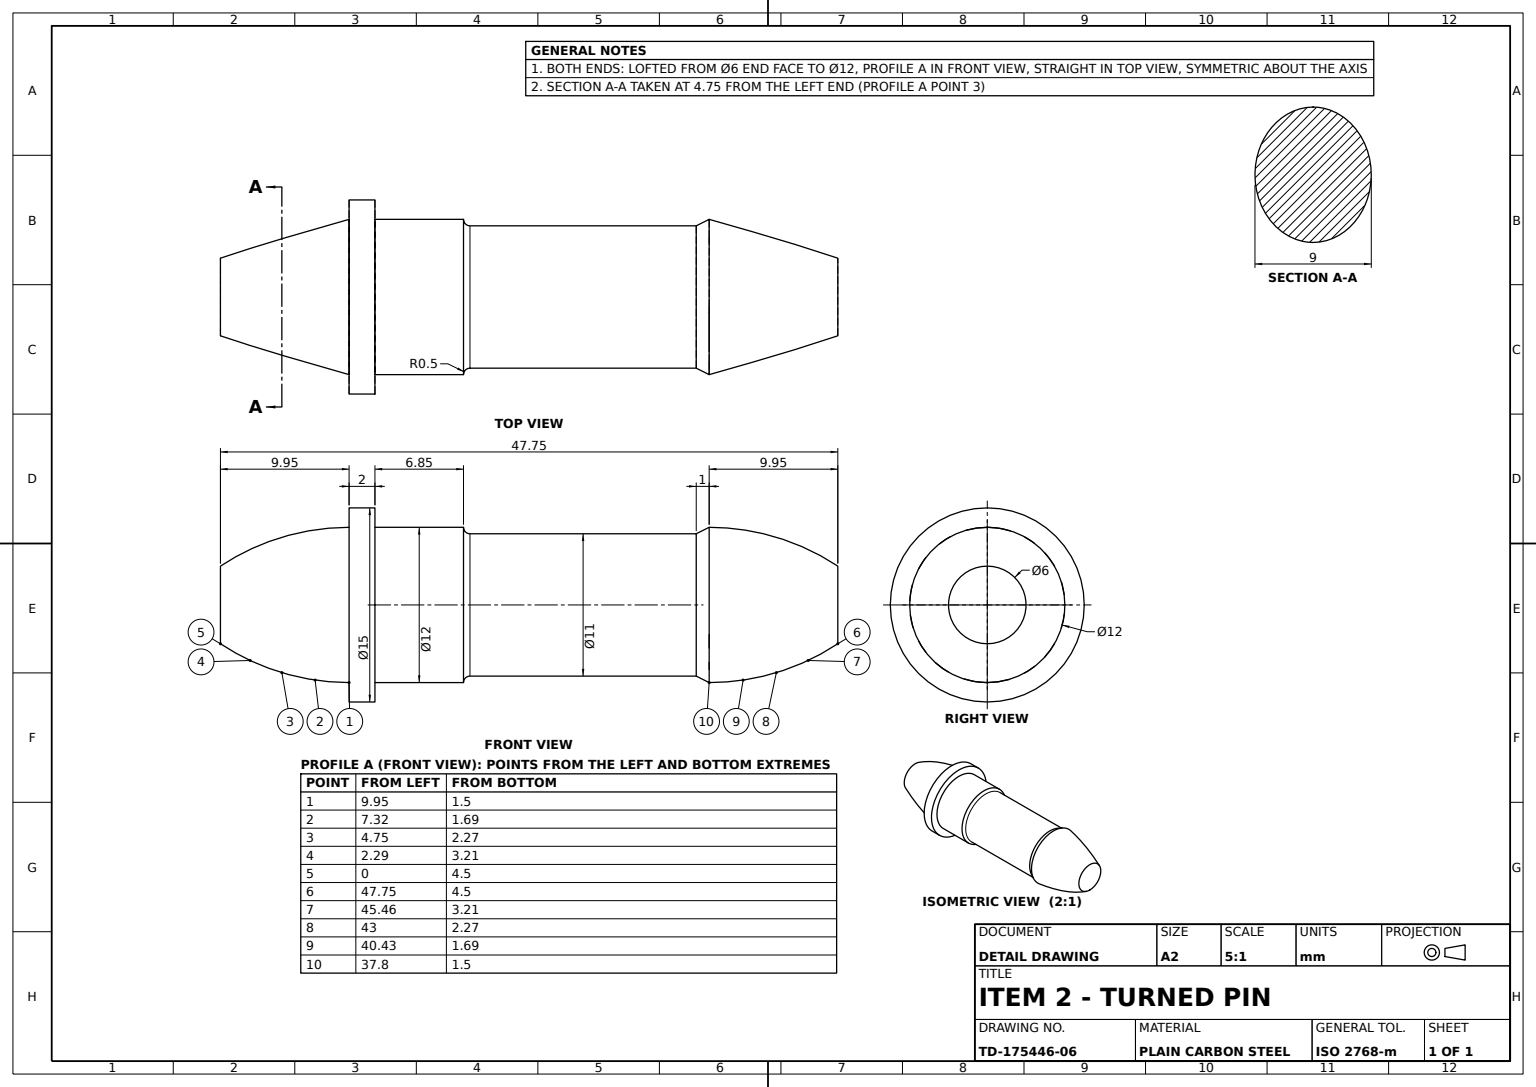
ISO-10303-21;
HEADER;
FILE_DESCRIPTION((''),'2;1');
FILE_NAME('','',(''),(''),'','','');
FILE_SCHEMA(('AUTOMOTIVE_DESIGN'));
ENDSEC;
DATA;
#1=APPLICATION_CONTEXT('');
#2=PRODUCT_CONTEXT('',#1,'mechanical');
#3=PRODUCT('','','',(#2));
#4=PRODUCT_DEFINITION_FORMATION('','',#3);
#5=PRODUCT_DEFINITION_CONTEXT('',#1,'design');
#6=PRODUCT_DEFINITION('','',#4,#5);
#7=PRODUCT_DEFINITION_SHAPE('','',#6);
#8=(LENGTH_UNIT()NAMED_UNIT(*)SI_UNIT(.MILLI.,.METRE.));
#9=(NAMED_UNIT(*)PLANE_ANGLE_UNIT()SI_UNIT($,.RADIAN.));
#10=(NAMED_UNIT(*)SI_UNIT($,.STERADIAN.)SOLID_ANGLE_UNIT());
#11=UNCERTAINTY_MEASURE_WITH_UNIT(LENGTH_MEASURE(1.E-05),#8,'distance_accuracy_value','');
#12=(GEOMETRIC_REPRESENTATION_CONTEXT(3)GLOBAL_UNCERTAINTY_ASSIGNED_CONTEXT((#11))GLOBAL_UNIT_ASSIGNED_CONTEXT((#8,#9,#10))REPRESENTATION_CONTEXT('',''));
#13=CARTESIAN_POINT('',(0.,11.95,7.5));
#14=VERTEX_POINT('',#13);
#15=CARTESIAN_POINT('',(0.,11.95,-7.5));
#16=VERTEX_POINT('',#15);
#17=CARTESIAN_POINT('',(0.,11.95,0.));
#18=DIRECTION('',(0.,1.,0.));
#19=DIRECTION('',(0.,0.,1.));
#20=AXIS2_PLACEMENT_3D('',#17,#18,#19);
#21=CIRCLE('',#20,7.5);
#22=EDGE_CURVE('',#14,#16,#21,.T.);
#23=ORIENTED_EDGE('',*,*,#22,.F.);
#24=CARTESIAN_POINT('',(0.,9.95,7.5));
#25=VERTEX_POINT('',#24);
#26=DIRECTION('',(0.,-1.,0.));
#27=VECTOR('',#26,1000.);
#28=LINE('',#13,#27);
#29=EDGE_CURVE('',#14,#25,#28,.T.);
#30=ORIENTED_EDGE('',*,*,#29,.T.);
#31=CARTESIAN_POINT('',(0.,9.95,-7.5));
#32=VERTEX_POINT('',#31);
#33=CARTESIAN_POINT('',(0.,9.95,0.));
#34=AXIS2_PLACEMENT_3D('',#33,#18,#19);
#35=CIRCLE('',#34,7.5);
#36=EDGE_CURVE('',#25,#32,#35,.T.);
#37=ORIENTED_EDGE('',*,*,#36,.T.);
#38=LINE('',#15,#27);
#39=EDGE_CURVE('',#16,#32,#38,.T.);
#40=ORIENTED_EDGE('',*,*,#39,.F.);
#41=EDGE_LOOP('',(#23,#30,#37,#40));
#42=FACE_OUTER_BOUND('',#41,.T.);
#43=DIRECTION('',(0.,0.,-1.));
#44=AXIS2_PLACEMENT_3D('',#17,#26,#43);
#45=CYLINDRICAL_SURFACE('',#44,7.5);
#46=ADVANCED_FACE('',(#42),#45,.T.);
#47=CARTESIAN_POINT('',(0.,11.95,6.));
#48=VERTEX_POINT('',#47);
#49=CARTESIAN_POINT('',(0.,11.95,-6.));
#50=VERTEX_POINT('',#49);
#51=CIRCLE('',#20,6.);
#52=EDGE_CURVE('',#48,#50,#51,.T.);
#53=ORIENTED_EDGE('',*,*,#52,.F.);
#54=EDGE_CURVE('',#50,#48,#51,.T.);
#55=ORIENTED_EDGE('',*,*,#54,.F.);
#56=EDGE_LOOP('',(#53,#55));
#57=FACE_BOUND('',#56,.T.);
#58=ORIENTED_EDGE('',*,*,#22,.T.);
#59=EDGE_CURVE('',#16,#14,#21,.T.);
#60=ORIENTED_EDGE('',*,*,#59,.T.);
#61=EDGE_LOOP('',(#58,#60));
#62=FACE_OUTER_BOUND('',#61,.T.);
#63=PLANE('',#20);
#64=ADVANCED_FACE('',(#57,#62),#63,.T.);
#65=CARTESIAN_POINT('',(0.,36.8,5.5));
#66=VERTEX_POINT('',#65);
#67=CARTESIAN_POINT('',(0.,19.3,5.5));
#68=VERTEX_POINT('',#67);
#69=LINE('',#65,#27);
#70=EDGE_CURVE('',#66,#68,#69,.T.);
#71=ORIENTED_EDGE('',*,*,#70,.T.);
#72=CARTESIAN_POINT('',(0.,19.3,-5.5));
#73=VERTEX_POINT('',#72);
#74=CARTESIAN_POINT('',(0.,19.3,0.));
#75=AXIS2_PLACEMENT_3D('',#74,#18,#19);
#76=CIRCLE('',#75,5.5);
#77=EDGE_CURVE('',#68,#73,#76,.T.);
#78=ORIENTED_EDGE('',*,*,#77,.T.);
#79=CARTESIAN_POINT('',(0.,36.8,-5.5));
#80=VERTEX_POINT('',#79);
#81=LINE('',#79,#27);
#82=EDGE_CURVE('',#80,#73,#81,.T.);
#83=ORIENTED_EDGE('',*,*,#82,.F.);
#84=CARTESIAN_POINT('',(0.,36.8,0.));
#85=AXIS2_PLACEMENT_3D('',#84,#18,#19);
#86=CIRCLE('',#85,5.5);
#87=EDGE_CURVE('',#66,#80,#86,.T.);
#88=ORIENTED_EDGE('',*,*,#87,.F.);
#89=EDGE_LOOP('',(#71,#78,#83,#88));
#90=FACE_OUTER_BOUND('',#89,.T.);
#91=AXIS2_PLACEMENT_3D('',#84,#26,#43);
#92=CYLINDRICAL_SURFACE('',#91,5.5);
#93=ADVANCED_FACE('',(#90),#92,.T.);
#94=ORIENTED_EDGE('',*,*,#82,.T.);
#95=EDGE_CURVE('',#73,#68,#76,.T.);
#96=ORIENTED_EDGE('',*,*,#95,.T.);
#97=ORIENTED_EDGE('',*,*,#70,.F.);
#98=EDGE_CURVE('',#80,#66,#86,.T.);
#99=ORIENTED_EDGE('',*,*,#98,.F.);
#100=EDGE_LOOP('',(#94,#96,#97,#99));
#101=FACE_OUTER_BOUND('',#100,.T.);
#102=ADVANCED_FACE('',(#101),#92,.T.);
#103=CARTESIAN_POINT('',(0.,18.8,6.));
#104=VERTEX_POINT('',#103);
#105=CARTESIAN_POINT('',(0.,19.3,6.));
#106=DIRECTION('',(-1.,0.,0.));
#107=AXIS2_PLACEMENT_3D('',#105,#106,#19);
#108=CIRCLE('',#107,0.5);
#109=EDGE_CURVE('',#68,#104,#108,.T.);
#110=ORIENTED_EDGE('',*,*,#109,.F.);
#111=ORIENTED_EDGE('',*,*,#95,.F.);
#112=CARTESIAN_POINT('',(0.,18.8,-6.));
#113=VERTEX_POINT('',#112);
#114=CARTESIAN_POINT('',(0.,19.3,-6.));
#115=DIRECTION('',(1.,0.,0.));
#116=AXIS2_PLACEMENT_3D('',#114,#115,#43);
#117=CIRCLE('',#116,0.5);
#118=EDGE_CURVE('',#73,#113,#117,.T.);
#119=ORIENTED_EDGE('',*,*,#118,.T.);
#120=CARTESIAN_POINT('',(0.,18.8,0.));
#121=AXIS2_PLACEMENT_3D('',#120,#18,#19);
#122=CIRCLE('',#121,6.);
#123=EDGE_CURVE('',#113,#104,#122,.T.);
#124=ORIENTED_EDGE('',*,*,#123,.T.);
#125=EDGE_LOOP('',(#110,#111,#119,#124));
#126=FACE_OUTER_BOUND('',#125,.T.);
#127=TOROIDAL_SURFACE('',#75,6.,0.5);
#128=ADVANCED_FACE('',(#126),#127,.F.);
#129=CARTESIAN_POINT('',(-3.,0.,0.));
#130=VERTEX_POINT('',#129);
#131=CARTESIAN_POINT('',(3.,0.,0.));
#132=VERTEX_POINT('',#131);
#133=CARTESIAN_POINT('',(0.,0.,0.));
#134=AXIS2_PLACEMENT_3D('',#133,#18,#19);
#135=CIRCLE('',#134,3.);
#136=EDGE_CURVE('',#130,#132,#135,.T.);
#137=ORIENTED_EDGE('',*,*,#136,.T.);
#138=CARTESIAN_POINT('',(6.,9.95,0.));
#139=VERTEX_POINT('',#138);
#140=CARTESIAN_POINT('',(6.000025,6.410631,0.));
#141=CARTESIAN_POINT('',(4.95646,2.949474,0.));
#142=B_SPLINE_CURVE_WITH_KNOTS('',3,(#138,#140,#141,#131),.UNSPECIFIED.,.F.,.F.,(4,4),(0.,1.),.UNSPECIFIED.);
#143=EDGE_CURVE('',#139,#132,#142,.T.);
#144=ORIENTED_EDGE('',*,*,#143,.F.);
#145=CARTESIAN_POINT('',(-6.,9.95,0.));
#146=VERTEX_POINT('',#145);
#147=CIRCLE('',#34,6.);
#148=EDGE_CURVE('',#146,#139,#147,.T.);
#149=ORIENTED_EDGE('',*,*,#148,.F.);
#150=CARTESIAN_POINT('',(-6.000025,6.410631,0.));
#151=CARTESIAN_POINT('',(-4.95646,2.949474,0.));
#152=B_SPLINE_CURVE_WITH_KNOTS('',3,(#145,#150,#151,#129),.UNSPECIFIED.,.F.,.F.,(4,4),(0.,1.),.UNSPECIFIED.);
#153=EDGE_CURVE('',#146,#130,#152,.T.);
#154=ORIENTED_EDGE('',*,*,#153,.T.);
#155=EDGE_LOOP('',(#137,#144,#149,#154));
#156=FACE_OUTER_BOUND('',#155,.T.);
#157=CARTESIAN_POINT('',(-6.,9.95,-0.785398));
#158=CARTESIAN_POINT('',(-6.000025,6.410631,-0.654498));
#159=CARTESIAN_POINT('',(-4.95646,2.949474,-0.523599));
#160=CARTESIAN_POINT('',(-3.,0.,-0.392699));
#161=CARTESIAN_POINT('',(-5.687979,9.95,-2.355842));
#162=CARTESIAN_POINT('',(-5.677499,6.410631,-1.963227));
#163=CARTESIAN_POINT('',(-4.688654,2.949474,-1.570612));
#164=CARTESIAN_POINT('',(-2.84397,0.,-1.177998));
#165=CARTESIAN_POINT('',(-4.353184,9.95,-4.353257));
#166=CARTESIAN_POINT('',(-4.33079,6.410631,-3.627716));
#167=CARTESIAN_POINT('',(-3.574621,2.949474,-2.902175));
#168=CARTESIAN_POINT('',(-2.176574,0.,-2.176634));
#169=CARTESIAN_POINT('',(-2.356027,9.95,-5.687748));
#170=CARTESIAN_POINT('',(-2.338359,6.410631,-4.739794));
#171=CARTESIAN_POINT('',(-1.929344,2.949474,-3.791841));
#172=CARTESIAN_POINT('',(-1.177994,0.,-2.843888));
#173=CARTESIAN_POINT('',(0.,9.95,-6.156445));
#174=CARTESIAN_POINT('',(0.,6.410631,-5.130367));
#175=CARTESIAN_POINT('',(0.,2.949474,-4.10429));
#176=CARTESIAN_POINT('',(0.,0.,-3.078212));
#177=CARTESIAN_POINT('',(2.356027,9.95,-5.687748));
#178=CARTESIAN_POINT('',(2.338359,6.410631,-4.739794));
#179=CARTESIAN_POINT('',(1.929344,2.949474,-3.791841));
#180=CARTESIAN_POINT('',(1.177994,0.,-2.843888));
#181=CARTESIAN_POINT('',(4.353184,9.95,-4.353257));
#182=CARTESIAN_POINT('',(4.33079,6.410631,-3.627716));
#183=CARTESIAN_POINT('',(3.574621,2.949474,-2.902175));
#184=CARTESIAN_POINT('',(2.176574,0.,-2.176634));
#185=CARTESIAN_POINT('',(5.687979,9.95,-2.355842));
#186=CARTESIAN_POINT('',(5.677499,6.410631,-1.963227));
#187=CARTESIAN_POINT('',(4.688654,2.949474,-1.570612));
#188=CARTESIAN_POINT('',(2.84397,0.,-1.177998));
#189=CARTESIAN_POINT('',(6.,9.95,-0.785398));
#190=CARTESIAN_POINT('',(6.000025,6.410631,-0.654498));
#191=CARTESIAN_POINT('',(4.95646,2.949474,-0.523599));
#192=CARTESIAN_POINT('',(3.,0.,-0.392699));
#193=CARTESIAN_POINT('',(6.,9.95,0.785398));
#194=CARTESIAN_POINT('',(6.000025,6.410631,0.654498));
#195=CARTESIAN_POINT('',(4.95646,2.949474,0.523599));
#196=CARTESIAN_POINT('',(3.,0.,0.392699));
#197=CARTESIAN_POINT('',(5.687979,9.95,2.355842));
#198=CARTESIAN_POINT('',(5.677499,6.410631,1.963227));
#199=CARTESIAN_POINT('',(4.688654,2.949474,1.570612));
#200=CARTESIAN_POINT('',(2.84397,0.,1.177998));
#201=CARTESIAN_POINT('',(4.353184,9.95,4.353257));
#202=CARTESIAN_POINT('',(4.33079,6.410631,3.627716));
#203=CARTESIAN_POINT('',(3.574621,2.949474,2.902175));
#204=CARTESIAN_POINT('',(2.176574,0.,2.176634));
#205=CARTESIAN_POINT('',(2.356027,9.95,5.687748));
#206=CARTESIAN_POINT('',(2.338359,6.410631,4.739794));
#207=CARTESIAN_POINT('',(1.929344,2.949474,3.791841));
#208=CARTESIAN_POINT('',(1.177994,0.,2.843888));
#209=CARTESIAN_POINT('',(0.,9.95,6.156445));
#210=CARTESIAN_POINT('',(0.,6.410631,5.130367));
#211=CARTESIAN_POINT('',(0.,2.949474,4.10429));
#212=CARTESIAN_POINT('',(0.,0.,3.078212));
#213=CARTESIAN_POINT('',(-2.356027,9.95,5.687748));
#214=CARTESIAN_POINT('',(-2.338359,6.410631,4.739794));
#215=CARTESIAN_POINT('',(-1.929344,2.949474,3.791841));
#216=CARTESIAN_POINT('',(-1.177994,0.,2.843888));
#217=CARTESIAN_POINT('',(-4.353184,9.95,4.353257));
#218=CARTESIAN_POINT('',(-4.33079,6.410631,3.627716));
#219=CARTESIAN_POINT('',(-3.574621,2.949474,2.902175));
#220=CARTESIAN_POINT('',(-2.176574,0.,2.176634));
#221=CARTESIAN_POINT('',(-5.687979,9.95,2.355842));
#222=CARTESIAN_POINT('',(-5.677499,6.410631,1.963227));
#223=CARTESIAN_POINT('',(-4.688654,2.949474,1.570612));
#224=CARTESIAN_POINT('',(-2.84397,0.,1.177998));
#225=CARTESIAN_POINT('',(-6.,9.95,0.785398));
#226=CARTESIAN_POINT('',(-6.000025,6.410631,0.654498));
#227=CARTESIAN_POINT('',(-4.95646,2.949474,0.523599));
#228=CARTESIAN_POINT('',(-3.,0.,0.392699));
#229=B_SPLINE_SURFACE_WITH_KNOTS('',3,3,((#145,#150,#151,#129),(#157,#158,#159,#160),(#161,#162,#163,#164),(#165,#166,#167,#168),(#169,#170,#171,#172),(#173,#174,#175,#176),(#177,#178,#179,#180),(#181,#182,#183,#184),(#185,#186,#187,#188),(#189,#190,#191,#192),(#193,#194,#195,#196),(#197,#198,#199,#200),(#201,#202,#203,#204),(#205,#206,#207,#208),(#209,#210,#211,#212),(#213,#214,#215,#216),(#217,#218,#219,#220),(#221,#222,#223,#224),(#225,#226,#227,#228),(#145,#150,#151,#129)),.UNSPECIFIED.,.T.,.F.,.F.,(4,1,1,1,1,1,1,1,2,1,1,1,1,1,1,1,4),(4,4),(0.,0.0625,0.125,0.1875,0.25,0.3125,0.375,0.4375,0.5,0.5625,0.625,0.6875,0.75,0.8125,0.875,0.9375,1.),(0.,1.),.UNSPECIFIED.);
#230=ADVANCED_FACE('',(#156),#229,.T.);
#231=ORIENTED_EDGE('',*,*,#143,.T.);
#232=EDGE_CURVE('',#132,#130,#135,.T.);
#233=ORIENTED_EDGE('',*,*,#232,.T.);
#234=ORIENTED_EDGE('',*,*,#153,.F.);
#235=EDGE_CURVE('',#139,#146,#147,.T.);
#236=ORIENTED_EDGE('',*,*,#235,.F.);
#237=EDGE_LOOP('',(#231,#233,#234,#236));
#238=FACE_OUTER_BOUND('',#237,.T.);
#239=ADVANCED_FACE('',(#238),#229,.T.);
#240=ORIENTED_EDGE('',*,*,#87,.T.);
#241=CARTESIAN_POINT('',(0.,37.800271,-6.000136));
#242=VERTEX_POINT('',#241);
#243=DIRECTION('',(0.,0.894427191,-0.447213595));
#244=VECTOR('',#243,1000.);
#245=LINE('',#79,#244);
#246=EDGE_CURVE('',#80,#242,#245,.T.);
#247=ORIENTED_EDGE('',*,*,#246,.T.);
#248=CARTESIAN_POINT('',(6.,37.8,0.));
#249=VERTEX_POINT('',#248);
#250=CARTESIAN_POINT('',(6.,37.8,-0.396106));
#251=CARTESIAN_POINT('',(5.96083,37.799345,-0.788083));
#252=CARTESIAN_POINT('',(5.805864,37.799586,-1.563958));
#253=CARTESIAN_POINT('',(5.691379,37.80042,-1.939901));
#254=CARTESIAN_POINT('',(5.466806,37.800439,-2.480886));
#255=CARTESIAN_POINT('',(5.383007,37.800219,-2.657661));
#256=CARTESIAN_POINT('',(5.197439,37.799868,-3.004071));
#257=CARTESIAN_POINT('',(5.09506,37.799736,-3.174509));
#258=CARTESIAN_POINT('',(4.766595,37.799721,-3.66508));
#259=CARTESIAN_POINT('',(4.51867,37.800321,-3.966961));
#260=CARTESIAN_POINT('',(3.96495,37.800289,-4.520413));
#261=CARTESIAN_POINT('',(3.655958,37.79972,-4.773424));
#262=CARTESIAN_POINT('',(3.004636,37.799744,-5.208062));
#263=CARTESIAN_POINT('',(2.660278,37.800276,-5.39254));
#264=CARTESIAN_POINT('',(2.114851,37.800271,-5.618519));
#265=CARTESIAN_POINT('',(1.927546,37.800108,-5.685407));
#266=CARTESIAN_POINT('',(1.551266,37.799856,-5.799254));
#267=CARTESIAN_POINT('',(1.361395,37.799765,-5.846652));
#268=CARTESIAN_POINT('',(0.786699,37.799773,-5.960901));
#269=CARTESIAN_POINT('',(0.395479,37.800271,-6.000136));
#270=B_SPLINE_CURVE_WITH_KNOTS('',3,(#248,#250,#251,#252,#253,#254,#255,#256,#257,#258,#259,#260,#261,#262,#263,#264,#265,#266,#267,#268,#269,#241),.UNSPECIFIED.,.F.,.F.,(4,2,2,2,2,2,2,2,2,2,4),(0.,0.001181769,0.002363539,0.002954424,0.003545308,0.004727078,0.005908847,0.007090617,0.007681501,0.008272386,0.009454155),.UNSPECIFIED.);
#271=EDGE_CURVE('',#249,#242,#270,.T.);
#272=ORIENTED_EDGE('',*,*,#271,.F.);
#273=CARTESIAN_POINT('',(0.,37.800271,6.000136));
#274=VERTEX_POINT('',#273);
#275=CARTESIAN_POINT('',(0.391395,37.800271,6.000136));
#276=CARTESIAN_POINT('',(0.780802,37.799774,5.961961));
#277=CARTESIAN_POINT('',(1.361889,37.799764,5.846609));
#278=CARTESIAN_POINT('',(1.554432,37.799857,5.798398));
#279=CARTESIAN_POINT('',(1.930162,37.80011,5.684511));
#280=CARTESIAN_POINT('',(2.114372,37.80027,5.618651));
#281=CARTESIAN_POINT('',(2.475504,37.800275,5.469161));
#282=CARTESIAN_POINT('',(2.652427,37.800116,5.385529));
#283=CARTESIAN_POINT('',(2.998941,37.799846,5.200386));
#284=CARTESIAN_POINT('',(3.169439,37.799737,5.098235));
#285=CARTESIAN_POINT('',(3.661542,37.799723,4.769396));
#286=CARTESIAN_POINT('',(3.963959,37.800287,4.521289));
#287=CARTESIAN_POINT('',(4.517933,37.800323,3.967811));
#288=CARTESIAN_POINT('',(4.771322,37.799716,3.658773));
#289=CARTESIAN_POINT('',(5.207048,37.799746,3.006486));
#290=CARTESIAN_POINT('',(5.391801,37.800449,2.661952));
#291=CARTESIAN_POINT('',(5.617869,37.800424,2.116788));
#292=CARTESIAN_POINT('',(5.684858,37.800172,1.92931));
#293=CARTESIAN_POINT('',(5.798959,37.799718,1.552159));
#294=CARTESIAN_POINT('',(5.846407,37.799521,1.361946));
#295=CARTESIAN_POINT('',(5.960742,37.79935,0.786529));
#296=CARTESIAN_POINT('',(6.,37.8,0.396444));
#297=B_SPLINE_CURVE_WITH_KNOTS('',3,(#273,#275,#276,#277,#278,#279,#280,#281,#282,#283,#284,#285,#286,#287,#288,#289,#290,#291,#292,#293,#294,#295,#296,#248),.UNSPECIFIED.,.F.,.F.,(4,2,2,2,2,2,2,2,2,2,2,4),(0.028375947,0.029558724,0.030150113,0.030741502,0.03133289,0.031924279,0.033107057,0.034289834,0.035472612,0.036064,0.036655389,0.037838166),.UNSPECIFIED.);
#298=EDGE_CURVE('',#274,#249,#297,.T.);
#299=ORIENTED_EDGE('',*,*,#298,.F.);
#300=DIRECTION('',(0.,0.894427191,0.447213595));
#301=VECTOR('',#300,1000.);
#302=LINE('',#65,#301);
#303=EDGE_CURVE('',#66,#274,#302,.T.);
#304=ORIENTED_EDGE('',*,*,#303,.F.);
#305=EDGE_LOOP('',(#240,#247,#272,#299,#304));
#306=FACE_OUTER_BOUND('',#305,.T.);
#307=CONICAL_SURFACE('',#85,5.5,0.463647609);
#308=ADVANCED_FACE('',(#306),#307,.T.);
#309=ORIENTED_EDGE('',*,*,#232,.F.);
#310=ORIENTED_EDGE('',*,*,#136,.F.);
#311=EDGE_LOOP('',(#309,#310));
#312=FACE_OUTER_BOUND('',#311,.T.);
#313=PLANE('',#134);
#314=ADVANCED_FACE('',(#312),#313,.F.);
#315=EDGE_CURVE('',#32,#25,#35,.T.);
#316=ORIENTED_EDGE('',*,*,#315,.F.);
#317=ORIENTED_EDGE('',*,*,#36,.F.);
#318=EDGE_LOOP('',(#316,#317));
#319=FACE_OUTER_BOUND('',#318,.T.);
#320=ORIENTED_EDGE('',*,*,#235,.T.);
#321=ORIENTED_EDGE('',*,*,#148,.T.);
#322=EDGE_LOOP('',(#320,#321));
#323=FACE_BOUND('',#322,.T.);
#324=PLANE('',#34);
#325=ADVANCED_FACE('',(#319,#323),#324,.F.);
#326=EDGE_CURVE('',#104,#113,#122,.T.);
#327=ORIENTED_EDGE('',*,*,#326,.T.);
#328=ORIENTED_EDGE('',*,*,#118,.F.);
#329=ORIENTED_EDGE('',*,*,#77,.F.);
#330=ORIENTED_EDGE('',*,*,#109,.T.);
#331=EDGE_LOOP('',(#327,#328,#329,#330));
#332=FACE_OUTER_BOUND('',#331,.T.);
#333=ADVANCED_FACE('',(#332),#127,.F.);
#334=ORIENTED_EDGE('',*,*,#39,.T.);
#335=ORIENTED_EDGE('',*,*,#315,.T.);
#336=ORIENTED_EDGE('',*,*,#29,.F.);
#337=ORIENTED_EDGE('',*,*,#59,.F.);
#338=EDGE_LOOP('',(#334,#335,#336,#337));
#339=FACE_OUTER_BOUND('',#338,.T.);
#340=ADVANCED_FACE('',(#339),#45,.T.);
#341=CARTESIAN_POINT('',(-6.,37.8,0.));
#342=VERTEX_POINT('',#341);
#343=CARTESIAN_POINT('',(-6.,37.8,0.391456));
#344=CARTESIAN_POINT('',(-5.960463,37.799348,0.788981));
#345=CARTESIAN_POINT('',(-5.807334,37.799582,1.557528));
#346=CARTESIAN_POINT('',(-5.694396,37.80041,1.931618));
#347=CARTESIAN_POINT('',(-5.468635,37.800444,2.476975));
#348=CARTESIAN_POINT('',(-5.383433,37.80022,2.65682));
#349=CARTESIAN_POINT('',(-5.197635,37.799868,3.00375));
#350=CARTESIAN_POINT('',(-5.096789,37.799738,3.171649));
#351=CARTESIAN_POINT('',(-4.770991,37.799718,3.659059));
#352=CARTESIAN_POINT('',(-4.522534,37.80032,3.963007));
#353=CARTESIAN_POINT('',(-3.962453,37.80029,4.523));
#354=CARTESIAN_POINT('',(-3.659317,37.799723,4.770807));
#355=CARTESIAN_POINT('',(-3.171758,37.799737,5.096723));
#356=CARTESIAN_POINT('',(-3.003709,37.799843,5.197655));
#357=CARTESIAN_POINT('',(-2.65624,37.800113,5.38367));
#358=CARTESIAN_POINT('',(-2.476492,37.800275,5.468752));
#359=CARTESIAN_POINT('',(-1.931843,37.800267,5.694209));
#360=CARTESIAN_POINT('',(-1.557858,37.799764,5.807368));
#361=CARTESIAN_POINT('',(-0.788514,37.799771,5.960766));
#362=CARTESIAN_POINT('',(-0.391202,37.800271,6.000136));
#363=B_SPLINE_CURVE_WITH_KNOTS('',3,(#341,#343,#344,#345,#346,#347,#348,#349,#350,#351,#352,#353,#354,#355,#356,#357,#358,#359,#360,#361,#362,#273),.UNSPECIFIED.,.F.,.F.,(4,2,2,2,2,2,2,2,2,2,4),(0.01891838,0.020100576,0.021282772,0.02187387,0.022464967,0.023647163,0.024829359,0.025420457,0.026011555,0.027193751,0.028375947),.UNSPECIFIED.);
#364=EDGE_CURVE('',#342,#274,#363,.T.);
#365=ORIENTED_EDGE('',*,*,#364,.F.);
#366=CARTESIAN_POINT('',(-0.3959,37.800271,-6.000136));
#367=CARTESIAN_POINT('',(-0.785591,37.799774,-5.961089));
#368=CARTESIAN_POINT('',(-1.361251,37.799765,-5.846696));
#369=CARTESIAN_POINT('',(-1.551646,37.799856,-5.799178));
#370=CARTESIAN_POINT('',(-1.929362,37.800109,-5.684818));
#371=CARTESIAN_POINT('',(-2.116584,37.800272,-5.617856));
#372=CARTESIAN_POINT('',(-2.66111,37.800274,-5.392084));
#373=CARTESIAN_POINT('',(-3.005742,37.799743,-5.20751));
#374=CARTESIAN_POINT('',(-3.658823,37.799722,-4.771325));
#375=CARTESIAN_POINT('',(-3.967566,37.800293,-4.51811));
#376=CARTESIAN_POINT('',(-4.520806,37.800317,-3.964512));
#377=CARTESIAN_POINT('',(-4.769144,37.799717,-3.661947));
#378=CARTESIAN_POINT('',(-5.208416,37.799746,-3.004524));
#379=CARTESIAN_POINT('',(-5.394292,37.800455,-2.656526));
#380=CARTESIAN_POINT('',(-5.618576,37.800421,-2.114788));
#381=CARTESIAN_POINT('',(-5.68446,37.800173,-1.930438));
#382=CARTESIAN_POINT('',(-5.798408,37.79972,-1.554165));
#383=CARTESIAN_POINT('',(-5.846642,37.79952,-1.361163));
#384=CARTESIAN_POINT('',(-5.961681,37.79935,-0.78099));
#385=CARTESIAN_POINT('',(-6.,37.8,-0.391731));
#386=B_SPLINE_CURVE_WITH_KNOTS('',3,(#241,#366,#367,#368,#369,#370,#371,#372,#373,#374,#375,#376,#377,#378,#379,#380,#381,#382,#383,#384,#385,#341),.UNSPECIFIED.,.F.,.F.,(4,2,2,2,2,2,2,2,2,2,4),(0.009454155,0.010637183,0.011228698,0.011820212,0.01300324,0.014186268,0.015369296,0.016552324,0.017143838,0.017735352,0.01891838),.UNSPECIFIED.);
#387=EDGE_CURVE('',#242,#342,#386,.T.);
#388=ORIENTED_EDGE('',*,*,#387,.F.);
#389=ORIENTED_EDGE('',*,*,#246,.F.);
#390=ORIENTED_EDGE('',*,*,#98,.T.);
#391=ORIENTED_EDGE('',*,*,#303,.T.);
#392=EDGE_LOOP('',(#365,#388,#389,#390,#391));
#393=FACE_OUTER_BOUND('',#392,.T.);
#394=ADVANCED_FACE('',(#393),#307,.T.);
#395=CARTESIAN_POINT('',(3.,47.75,0.));
#396=VERTEX_POINT('',#395);
#397=CARTESIAN_POINT('',(-3.,47.75,0.));
#398=VERTEX_POINT('',#397);
#399=CARTESIAN_POINT('',(0.,47.75,0.));
#400=AXIS2_PLACEMENT_3D('',#399,#18,#19);
#401=CIRCLE('',#400,3.);
#402=EDGE_CURVE('',#396,#398,#401,.T.);
#403=ORIENTED_EDGE('',*,*,#402,.T.);
#404=EDGE_CURVE('',#398,#396,#401,.T.);
#405=ORIENTED_EDGE('',*,*,#404,.T.);
#406=EDGE_LOOP('',(#403,#405));
#407=FACE_OUTER_BOUND('',#406,.T.);
#408=PLANE('',#400);
#409=ADVANCED_FACE('',(#407),#408,.T.);
#410=ORIENTED_EDGE('',*,*,#402,.F.);
#411=CARTESIAN_POINT('',(4.95646,44.800526,0.));
#412=CARTESIAN_POINT('',(6.000025,41.339369,0.));
#413=B_SPLINE_CURVE_WITH_KNOTS('',3,(#395,#411,#412,#248),.UNSPECIFIED.,.F.,.F.,(4,4),(0.,1.),.UNSPECIFIED.);
#414=EDGE_CURVE('',#396,#249,#413,.T.);
#415=ORIENTED_EDGE('',*,*,#414,.T.);
#416=ORIENTED_EDGE('',*,*,#271,.T.);
#417=ORIENTED_EDGE('',*,*,#387,.T.);
#418=CARTESIAN_POINT('',(-4.95646,44.800526,0.));
#419=CARTESIAN_POINT('',(-6.000025,41.339369,0.));
#420=B_SPLINE_CURVE_WITH_KNOTS('',3,(#397,#418,#419,#341),.UNSPECIFIED.,.F.,.F.,(4,4),(0.,1.),.UNSPECIFIED.);
#421=EDGE_CURVE('',#398,#342,#420,.T.);
#422=ORIENTED_EDGE('',*,*,#421,.F.);
#423=EDGE_LOOP('',(#410,#415,#416,#417,#422));
#424=FACE_OUTER_BOUND('',#423,.T.);
#425=CARTESIAN_POINT('',(-6.,37.764606,0.));
#426=CARTESIAN_POINT('',(-6.,37.729213,0.));
#427=CARTESIAN_POINT('',(-5.999999,37.693819,0.));
#428=CARTESIAN_POINT('',(-3.,47.75,-0.392699));
#429=CARTESIAN_POINT('',(-4.95646,44.800526,-0.523599));
#430=CARTESIAN_POINT('',(-6.000025,41.339369,-0.654498));
#431=CARTESIAN_POINT('',(-6.,37.8,-0.785398));
#432=CARTESIAN_POINT('',(-6.,37.764606,-0.786707));
#433=CARTESIAN_POINT('',(-6.,37.729213,-0.788016));
#434=CARTESIAN_POINT('',(-5.999999,37.693819,-0.789325));
#435=CARTESIAN_POINT('',(-2.84397,47.75,-1.177998));
#436=CARTESIAN_POINT('',(-4.688654,44.800526,-1.570612));
#437=CARTESIAN_POINT('',(-5.677499,41.339369,-1.963227));
#438=CARTESIAN_POINT('',(-5.687979,37.8,-2.355842));
#439=CARTESIAN_POINT('',(-5.688083,37.764606,-2.359768));
#440=CARTESIAN_POINT('',(-5.688188,37.729213,-2.363694));
#441=CARTESIAN_POINT('',(-5.688293,37.693819,-2.36762));
#442=CARTESIAN_POINT('',(-2.176574,47.75,-2.176634));
#443=CARTESIAN_POINT('',(-3.574621,44.800526,-2.902175));
#444=CARTESIAN_POINT('',(-4.33079,41.339369,-3.627716));
#445=CARTESIAN_POINT('',(-4.353184,37.8,-4.353257));
#446=CARTESIAN_POINT('',(-4.353408,37.764606,-4.360512));
#447=CARTESIAN_POINT('',(-4.353632,37.729213,-4.367767));
#448=CARTESIAN_POINT('',(-4.353856,37.693819,-4.375023));
#449=CARTESIAN_POINT('',(-1.177994,47.75,-2.843888));
#450=CARTESIAN_POINT('',(-1.929344,44.800526,-3.791841));
#451=CARTESIAN_POINT('',(-2.338359,41.339369,-4.739794));
#452=CARTESIAN_POINT('',(-2.356027,37.8,-5.687748));
#453=CARTESIAN_POINT('',(-2.356204,37.764606,-5.697227));
#454=CARTESIAN_POINT('',(-2.35638,37.729213,-5.706707));
#455=CARTESIAN_POINT('',(-2.356557,37.693819,-5.716186));
#456=CARTESIAN_POINT('',(0.,47.75,-3.078212));
#457=CARTESIAN_POINT('',(0.,44.800526,-4.10429));
#458=CARTESIAN_POINT('',(0.,41.339369,-5.130367));
#459=CARTESIAN_POINT('',(0.,37.8,-6.156445));
#460=CARTESIAN_POINT('',(0.,37.764606,-6.166705));
#461=CARTESIAN_POINT('',(0.,37.729213,-6.176966));
#462=CARTESIAN_POINT('',(0.,37.693819,-6.187227));
#463=CARTESIAN_POINT('',(1.177994,47.75,-2.843888));
#464=CARTESIAN_POINT('',(1.929344,44.800526,-3.791841));
#465=CARTESIAN_POINT('',(2.338359,41.339369,-4.739794));
#466=CARTESIAN_POINT('',(2.356027,37.8,-5.687748));
#467=CARTESIAN_POINT('',(2.356204,37.764606,-5.697227));
#468=CARTESIAN_POINT('',(2.35638,37.729213,-5.706707));
#469=CARTESIAN_POINT('',(2.356557,37.693819,-5.716186));
#470=CARTESIAN_POINT('',(2.176574,47.75,-2.176634));
#471=CARTESIAN_POINT('',(3.574621,44.800526,-2.902175));
#472=CARTESIAN_POINT('',(4.33079,41.339369,-3.627716));
#473=CARTESIAN_POINT('',(4.353184,37.8,-4.353257));
#474=CARTESIAN_POINT('',(4.353408,37.764606,-4.360512));
#475=CARTESIAN_POINT('',(4.353632,37.729213,-4.367767));
#476=CARTESIAN_POINT('',(4.353856,37.693819,-4.375023));
#477=CARTESIAN_POINT('',(2.84397,47.75,-1.177998));
#478=CARTESIAN_POINT('',(4.688654,44.800526,-1.570612));
#479=CARTESIAN_POINT('',(5.677499,41.339369,-1.963227));
#480=CARTESIAN_POINT('',(5.687979,37.8,-2.355842));
#481=CARTESIAN_POINT('',(5.688083,37.764606,-2.359768));
#482=CARTESIAN_POINT('',(5.688188,37.729213,-2.363694));
#483=CARTESIAN_POINT('',(5.688293,37.693819,-2.36762));
#484=CARTESIAN_POINT('',(3.,47.75,-0.392699));
#485=CARTESIAN_POINT('',(4.95646,44.800526,-0.523599));
#486=CARTESIAN_POINT('',(6.000025,41.339369,-0.654498));
#487=CARTESIAN_POINT('',(6.,37.8,-0.785398));
#488=CARTESIAN_POINT('',(6.,37.764606,-0.786707));
#489=CARTESIAN_POINT('',(6.,37.729213,-0.788016));
#490=CARTESIAN_POINT('',(5.999999,37.693819,-0.789325));
#491=CARTESIAN_POINT('',(3.,47.75,0.392699));
#492=CARTESIAN_POINT('',(4.95646,44.800526,0.523599));
#493=CARTESIAN_POINT('',(6.000025,41.339369,0.654498));
#494=CARTESIAN_POINT('',(6.,37.8,0.785398));
#495=CARTESIAN_POINT('',(6.,37.764606,0.786707));
#496=CARTESIAN_POINT('',(6.,37.729213,0.788016));
#497=CARTESIAN_POINT('',(5.999999,37.693819,0.789325));
#498=CARTESIAN_POINT('',(2.84397,47.75,1.177998));
#499=CARTESIAN_POINT('',(4.688654,44.800526,1.570612));
#500=CARTESIAN_POINT('',(5.677499,41.339369,1.963227));
#501=CARTESIAN_POINT('',(5.687979,37.8,2.355842));
#502=CARTESIAN_POINT('',(5.688083,37.764606,2.359768));
#503=CARTESIAN_POINT('',(5.688188,37.729213,2.363694));
#504=CARTESIAN_POINT('',(5.688293,37.693819,2.36762));
#505=CARTESIAN_POINT('',(2.176574,47.75,2.176634));
#506=CARTESIAN_POINT('',(3.574621,44.800526,2.902175));
#507=CARTESIAN_POINT('',(4.33079,41.339369,3.627716));
#508=CARTESIAN_POINT('',(4.353184,37.8,4.353257));
#509=CARTESIAN_POINT('',(4.353408,37.764606,4.360512));
#510=CARTESIAN_POINT('',(4.353632,37.729213,4.367767));
#511=CARTESIAN_POINT('',(4.353856,37.693819,4.375023));
#512=CARTESIAN_POINT('',(1.177994,47.75,2.843888));
#513=CARTESIAN_POINT('',(1.929344,44.800526,3.791841));
#514=CARTESIAN_POINT('',(2.338359,41.339369,4.739794));
#515=CARTESIAN_POINT('',(2.356027,37.8,5.687748));
#516=CARTESIAN_POINT('',(2.356204,37.764606,5.697227));
#517=CARTESIAN_POINT('',(2.35638,37.729213,5.706707));
#518=CARTESIAN_POINT('',(2.356557,37.693819,5.716186));
#519=CARTESIAN_POINT('',(0.,47.75,3.078212));
#520=CARTESIAN_POINT('',(0.,44.800526,4.10429));
#521=CARTESIAN_POINT('',(0.,41.339369,5.130367));
#522=CARTESIAN_POINT('',(0.,37.8,6.156445));
#523=CARTESIAN_POINT('',(0.,37.764606,6.166705));
#524=CARTESIAN_POINT('',(0.,37.729213,6.176966));
#525=CARTESIAN_POINT('',(0.,37.693819,6.187227));
#526=CARTESIAN_POINT('',(-1.177994,47.75,2.843888));
#527=CARTESIAN_POINT('',(-1.929344,44.800526,3.791841));
#528=CARTESIAN_POINT('',(-2.338359,41.339369,4.739794));
#529=CARTESIAN_POINT('',(-2.356027,37.8,5.687748));
#530=CARTESIAN_POINT('',(-2.356204,37.764606,5.697227));
#531=CARTESIAN_POINT('',(-2.35638,37.729213,5.706707));
#532=CARTESIAN_POINT('',(-2.356557,37.693819,5.716186));
#533=CARTESIAN_POINT('',(-2.176574,47.75,2.176634));
#534=CARTESIAN_POINT('',(-3.574621,44.800526,2.902175));
#535=CARTESIAN_POINT('',(-4.33079,41.339369,3.627716));
#536=CARTESIAN_POINT('',(-4.353184,37.8,4.353257));
#537=CARTESIAN_POINT('',(-4.353408,37.764606,4.360512));
#538=CARTESIAN_POINT('',(-4.353632,37.729213,4.367767));
#539=CARTESIAN_POINT('',(-4.353856,37.693819,4.375023));
#540=CARTESIAN_POINT('',(-2.84397,47.75,1.177998));
#541=CARTESIAN_POINT('',(-4.688654,44.800526,1.570612));
#542=CARTESIAN_POINT('',(-5.677499,41.339369,1.963227));
#543=CARTESIAN_POINT('',(-5.687979,37.8,2.355842));
#544=CARTESIAN_POINT('',(-5.688083,37.764606,2.359768));
#545=CARTESIAN_POINT('',(-5.688188,37.729213,2.363694));
#546=CARTESIAN_POINT('',(-5.688293,37.693819,2.36762));
#547=CARTESIAN_POINT('',(-3.,47.75,0.392699));
#548=CARTESIAN_POINT('',(-4.95646,44.800526,0.523599));
#549=CARTESIAN_POINT('',(-6.000025,41.339369,0.654498));
#550=CARTESIAN_POINT('',(-6.,37.8,0.785398));
#551=CARTESIAN_POINT('',(-6.,37.764606,0.786707));
#552=CARTESIAN_POINT('',(-6.,37.729213,0.788016));
#553=CARTESIAN_POINT('',(-5.999999,37.693819,0.789325));
#554=B_SPLINE_SURFACE_WITH_KNOTS('',3,3,((#397,#418,#419,#341,#425,#426,#427),(#428,#429,#430,#431,#432,#433,#434),(#435,#436,#437,#438,#439,#440,#441),(#442,#443,#444,#445,#446,#447,#448),(#449,#450,#451,#452,#453,#454,#455),(#456,#457,#458,#459,#460,#461,#462),(#463,#464,#465,#466,#467,#468,#469),(#470,#471,#472,#473,#474,#475,#476),(#477,#478,#479,#480,#481,#482,#483),(#484,#485,#486,#487,#488,#489,#490),(#491,#492,#493,#494,#495,#496,#497),(#498,#499,#500,#501,#502,#503,#504),(#505,#506,#507,#508,#509,#510,#511),(#512,#513,#514,#515,#516,#517,#518),(#519,#520,#521,#522,#523,#524,#525),(#526,#527,#528,#529,#530,#531,#532),(#533,#534,#535,#536,#537,#538,#539),(#540,#541,#542,#543,#544,#545,#546),(#547,#548,#549,#550,#551,#552,#553),(#397,#418,#419,#341,#425,#426,#427)),.UNSPECIFIED.,.T.,.F.,.F.,(4,1,1,1,1,1,1,1,2,1,1,1,1,1,1,1,4),(4,3,4),(0.,0.0625,0.125,0.1875,0.25,0.3125,0.375,0.4375,0.5,0.5625,0.625,0.6875,0.75,0.8125,0.875,0.9375,1.),(0.,1.,1.01),.UNSPECIFIED.);
#555=ADVANCED_FACE('',(#424),#554,.T.);
#556=ORIENTED_EDGE('',*,*,#52,.T.);
#557=LINE('',#112,#27);
#558=EDGE_CURVE('',#113,#50,#557,.T.);
#559=ORIENTED_EDGE('',*,*,#558,.F.);
#560=ORIENTED_EDGE('',*,*,#326,.F.);
#561=LINE('',#103,#27);
#562=EDGE_CURVE('',#104,#48,#561,.T.);
#563=ORIENTED_EDGE('',*,*,#562,.T.);
#564=EDGE_LOOP('',(#556,#559,#560,#563));
#565=FACE_OUTER_BOUND('',#564,.T.);
#566=AXIS2_PLACEMENT_3D('',#120,#26,#43);
#567=CYLINDRICAL_SURFACE('',#566,6.);
#568=ADVANCED_FACE('',(#565),#567,.T.);
#569=ORIENTED_EDGE('',*,*,#123,.F.);
#570=ORIENTED_EDGE('',*,*,#558,.T.);
#571=ORIENTED_EDGE('',*,*,#54,.T.);
#572=ORIENTED_EDGE('',*,*,#562,.F.);
#573=EDGE_LOOP('',(#569,#570,#571,#572));
#574=FACE_OUTER_BOUND('',#573,.T.);
#575=ADVANCED_FACE('',(#574),#567,.T.);
#576=ORIENTED_EDGE('',*,*,#421,.T.);
#577=ORIENTED_EDGE('',*,*,#364,.T.);
#578=ORIENTED_EDGE('',*,*,#298,.T.);
#579=ORIENTED_EDGE('',*,*,#414,.F.);
#580=ORIENTED_EDGE('',*,*,#404,.F.);
#581=EDGE_LOOP('',(#576,#577,#578,#579,#580));
#582=FACE_OUTER_BOUND('',#581,.T.);
#583=ADVANCED_FACE('',(#582),#554,.T.);
#584=CLOSED_SHELL('',(#46,#64,#93,#102,#128,#230,#239,#308,#314,#325,#333,#340,#394,#409,#555,#568,#575,#583));
#585=MANIFOLD_SOLID_BREP('',#584);
#586=ADVANCED_BREP_SHAPE_REPRESENTATION('',(#585),#12);
#587=SHAPE_DEFINITION_REPRESENTATION(#7,#586);
ENDSEC;
END-ISO-10303-21;
